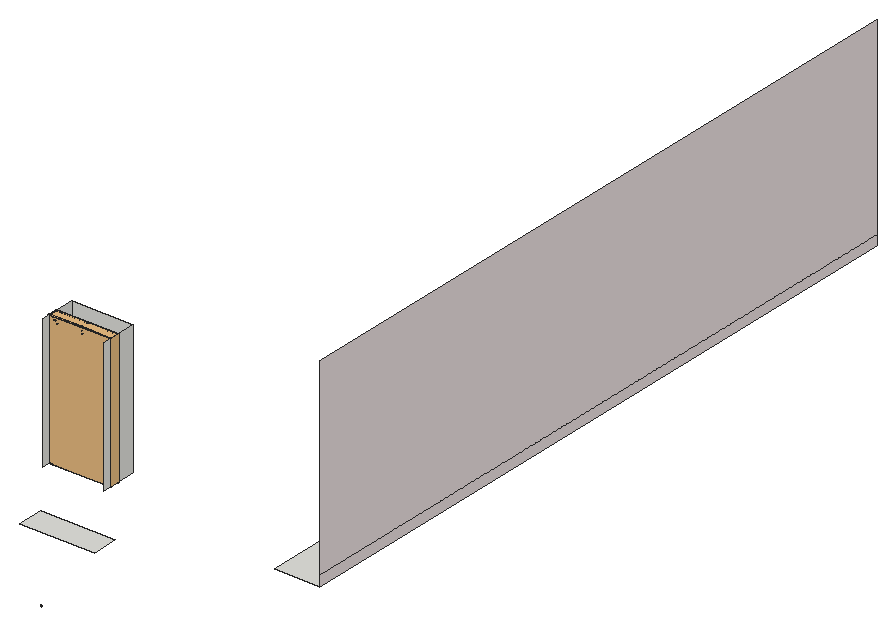
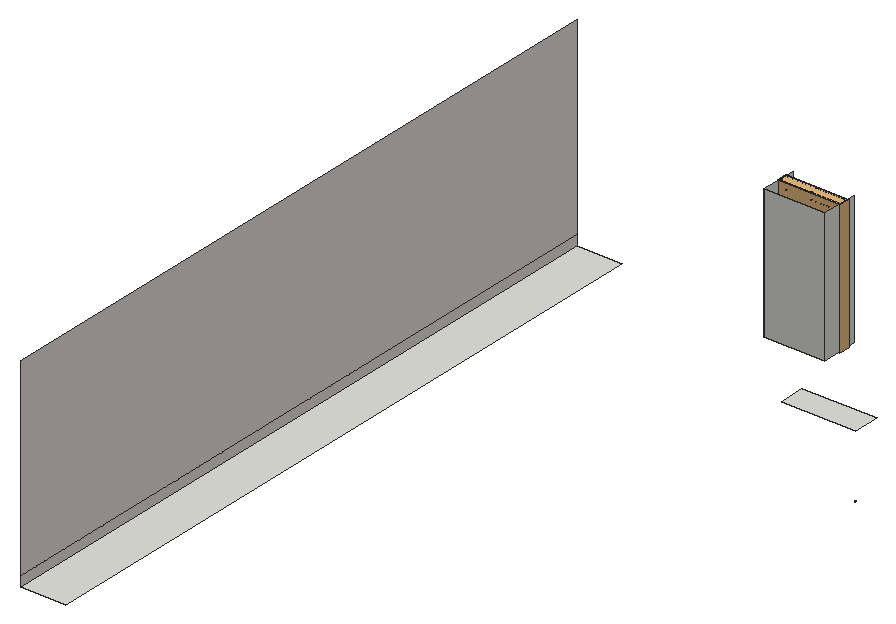
# SketchUp Ruby script. Lengths in inches.
U = 1.inch
M = Sketchup.active_model
def pt(a) = Geom::Point3d.new(a.map { |v| v * U })
def face(e, loops, mat)
  f = e.add_face(loops[0].map { |a| pt(a) })
  loops[1..].each { |l| e.add_face(l.map { |a| pt(a) }).erase! }
  f.material = f.back_material = mat if mat
  f
end
# faces: each face lists its corners as indices into pts; further lists are holes
def faces(e, pts, list, mat = nil) = list.each { |f| face(e, (f[0].is_a?(Array) ? f : [f]).map { |l| l.map { |i| pts[i] } }, mat) }
# xy, xz, yz: faces in a plane at the given z, y or x. An outline is a flat list of corners, or four numbers for a rectangle; further outlines are holes
def ring(l) = l.size == 4 ? [[l[0], l[1]], [l[2], l[1]], [l[2], l[3]], [l[0], l[3]]] : l.each_slice(2).to_a
def flat(e, list, mat, &to3) = list.each { |f| face(e, (f[0].is_a?(Array) ? f : [f]).map { |l| ring(l).map { |u, v| to3.(u, v) } }, mat) }
def xy(e, z, list, mat = nil) = flat(e, list, mat) { |x, y| [x, y, z] }
def xz(e, y, list, mat = nil) = flat(e, list, mat) { |x, z| [x, y, z] }
def yz(e, x, list, mat = nil) = flat(e, list, mat) { |y, z| [x, y, z] }
def lines(e, pts, list) = list.each { |a, b| e.add_line(pt(pts[a]), pt(pts[b])) }
# prism: a flat outline (further loops are holes) pulled along v
def prism(e, loops, v, mat = nil)
  f = face(e, loops, mat); d = Geom::Vector3d.new(v.map { |x| x * U })
  f.pushpull(f.normal.samedirection?(d) ? d.length : -d.length)
end
def box(e, o, s, mat = nil) = prism(e, [[o, [o[0] + s[0], o[1], o[2]], [o[0] + s[0], o[1] + s[1], o[2]], [o[0], o[1] + s[1], o[2]]]], [0, 0, s[2]], mat)
def at(x, y, z, deg = 0) = Geom::Transformation.translation(pt([x, y, z])) * Geom::Transformation.rotation(ORIGIN, Z_AXIS, deg.degrees)
def axes(o, x, y, z) = Geom::Transformation.new([*x, 0, *y, 0, *z, 0, *pt(o).to_a, 1])
def part(name) = M.definitions.add(name)
# library, detail: a bought-in or finely detailed component or shape, given as its bounding box
def library(name, o, s) = part(name).tap { |d| box(d.entities, o, s) }
def detail(e, o, s) = box(e.add_group.entities, o, s)
def put(e, d, t, mat = nil) = e.add_instance(d, t).tap { |i| i.material = mat if mat }
def group(e, t, mat = nil) = e.add_group.tap { |g| g.transformation = t; g.material = mat if mat }.entities
root = M.entities
M.materials.add("Generic\#9").color = [233, 223, 223]
M.materials.add("Material \#0").color = [86, 53, 35]
M.materials.add("Material \#1").color = [140, 140, 140]
c1 = part("3DGeom~19_Defintion")
xy(c1.entities,0,[[-6.28,-215.79,-994.45,-208.55,-13.52,-208.55],[-994.45,-215.79,-994.45,-208.55,-6.28,-215.79],[-6.28,-215.79,-13.52,-208.55,-13.52,0],[-6.28,-215.79,-13.52,0,-6.28,0],[-13.52,0,-13.52,208.55,-6.28,215.79],
  [-13.52,0,-6.28,215.79,-6.28,0],[-994.45,208.55,-6.28,215.79,-13.52,208.55],[-994.45,208.55,-994.45,215.79,-6.28,215.79]],"Material \#0")
p = [[-13.52,-208.55,0],[-994.45,-208.55,0],[-994.45,-207.81,0.07],[-14.25,-207.81,0.07],[-13.52,-208.55,0],[-14.25,-207.81,0.07],
  [-14.25,0,0.07],[-13.52,0,0],[-13.52,208.55,0],[-14.25,207.81,0.07],[-13.52,208.55,0],[-14.25,207.81,0.07],
  [-994.45,207.81,0.07],[-994.45,208.55,0],[-994.45,-207.21,0.27],[-994.45,-207.21,0.27],[-14.86,-207.21,0.27],[-14.86,-207.21,0.27],
  [-14.86,0,0.27],[-14.86,0,0.27],[-14.86,0,0.27],[-14.86,0,0.27],[-14.86,207.21,0.27],[-14.86,207.21,0.27],
  [-994.45,207.21,0.27],[-994.45,207.21,0.27],[-14.86,-207.21,0.27],[-994.45,-207.21,0.27],[-994.45,-206.74,0.6],[-15.33,-206.74,0.6],
  [-14.86,-207.21,0.27],[-15.33,-206.74,0.6],[-15.33,0,0.6],[-14.86,0,0.27],[-14.86,207.21,0.27],[-15.33,206.74,0.6],
  [-14.86,207.21,0.27],[-15.33,206.74,0.6],[-994.45,206.74,0.6],[-994.45,207.21,0.27],[-994.45,-206.4,1.07],[-15.66,-206.4,1.07],
  [-15.66,-206.4,1.07],[-15.66,0,1.07],[-15.66,206.4,1.07],[-15.66,206.4,1.07],[-994.45,206.4,1.07],[-994.45,-206.2,1.68],
  [-15.86,-206.2,1.68],[-15.86,-206.2,1.68],[-15.86,0,1.68],[-15.86,206.2,1.68],[-15.86,206.2,1.68],[-994.45,206.2,1.68],
  [-994.45,-206.13,2.41],[-15.93,-206.13,2.41],[-15.93,-206.13,2.41],[-15.93,0,2.41],[-15.93,206.13,2.41],[-15.93,206.13,2.41],
  [-994.45,206.13,2.41],[-994.45,-206.13,71.16],[-994.45,-206.22,71.59],[-15.79,-206.28,71.53],[-15.79,-206.28,71.53],[-15.84,0,71.59],
  [-15.93,0,71.16],[-15.79,206.28,71.53],[-15.79,206.28,71.53],[-994.45,206.22,71.59],[-994.45,206.13,71.16],[-15.79,-206.28,71.53],
  [-994.45,-206.48,71.84],[-994.45,-206.9,71.93],[-15.16,-206.9,71.93],[-15.79,-206.28,71.53],[-15.79,-206.28,71.53],[-15.16,-206.9,71.93],
  [-15.16,0,71.93],[-994.45,-206.48,71.84],[-15.59,0,71.84],[-15.79,-206.28,71.53],[-15.59,0,71.84],[-15.79,206.28,71.53],
  [-15.16,206.9,71.93],[-15.59,0,71.84],[-15.79,206.28,71.53],[-994.45,206.48,71.84],[-15.79,206.28,71.53],[-15.16,206.9,71.93],
  [-994.45,206.9,71.93],[-994.45,206.48,71.84],[-15.79,206.28,71.53],[-994.45,-227.27,72.01],[5.41,-227.47,72.33],[4.78,-226.84,71.93],
  [4.78,-226.84,71.93],[5.41,-227.47,72.33],[5.21,0,72.01],[-994.45,-226.84,71.93],[-994.45,-227.27,72.01],[5.21,0,72.01],
  [4.78,0,71.93],[4.78,226.84,71.93],[5.21,0,72.01],[5.21,0,72.01],[5.41,227.47,72.33],[4.78,226.84,71.93],
  [5.41,227.47,72.33],[-994.45,227.27,72.01],[-994.45,227.27,72.01],[-994.45,226.84,71.93],[-994.45,-227.27,72.01],[-994.45,-227.53,72.27],
  [5.41,-227.47,72.33],[5.41,-227.47,72.33],[5.47,0,72.27],[5.21,0,72.01],[5.41,227.47,72.33],[5.41,227.47,72.33],
  [-994.45,227.53,72.27],[-994.45,227.27,72.01],[-994.45,-227.61,72.7],[-994.45,-227.61,74.4375],[-994.45,-227.61,74.4375],[5.55,-227.61,74.4375],
  [5.55,-227.61,74.4375],[5.55,0,74.4375],[5.55,0,72.7],[5.55,227.61,74.4375],[5.55,227.61,74.4375],[-994.45,227.61,74.4375],
  [-994.45,227.61,74.4375],[-994.45,227.61,72.7]]
faces(c1.entities,p,[[0,1,2],[2,3,0],[4,5,6],[6,7,4],[8,7,6],[6,9,8],[10,11,12],[12,13,10],
  [3,2,14],[15,16,3],[5,17,18],[19,6,5],[9,6,20],[21,22,9],[11,23,24],[25,12,11],
  [26,27,28],[28,29,26],[30,31,32],[32,33,30],[34,33,32],[32,35,34],[36,37,38],[38,39,36],
  [29,28,40],[40,41,29],[31,42,43],[43,32,31],[35,32,43],[43,44,35],[37,45,46],[46,38,37],
  [41,40,47],[47,48,41],[42,49,50],[50,43,42],[44,43,50],[50,51,44],[45,52,53],[53,46,45],
  [48,47,54],[54,55,48],[49,56,57],[57,50,49],[51,50,57],[57,58,51],[52,59,60],[60,53,52],
  [61,62,63],[64,65,66],[66,65,67],[68,69,70],[71,72,73],[73,74,75],[76,77,78],[62,79,63],
  [78,80,76],[81,82,65],[83,80,78],[78,84,83],[65,85,86],[68,87,69],[88,89,90],[90,91,92],
  [93,94,95],[96,97,98],[95,99,100],[101,102,96],[103,102,104],[105,106,103],[107,108,109],[110,111,107],
  [112,113,114],[115,116,117],[117,116,118],[119,120,121],[114,122,123],[124,125,114],[113,122,114],[115,126,127],
  [127,128,115],[115,128,116],[118,128,127],[127,129,118],[116,128,118],[119,130,131],[132,133,119],[119,133,120]],"Material \#0")
c2 = part("3DGeom~15_Defintion")
xy(c2.entities,0,[[-961.58,-251.9,-958.5,-248.8125,-961.58,-237.8],[-961.58,-251.9,28.8,-248.8125,-958.5,-248.8125],[-961.58,-251.9,36.25,-251.9,28.8,-248.8125],[36.25,-251.9,19.98,-239.99,28.8,-248.8125],[36.25,-251.9,22.16,-237.8,19.98,-239.99],
  [-958.5,-248.8125,-958.5,-237.8,-961.58,-237.8],[19.98,-239.99,22.16,-237.8,3.36,-223.37],[-958.5,-237.8,-958.5,-223.37,-961.58,-220.28],[-961.58,-237.8,-958.5,-237.8,-961.58,-220.28],[22.16,-237.8,4.64,-220.28,3.36,-223.37],
  [-958.5,-223.37,4.64,-220.28,-961.58,-220.28],[-958.5,-223.37,3.36,-223.37,4.64,-220.28],[5.29,-219.63,8.375,-218.35,5.29,0],[8.375,-218.35,8.375,0,5.29,0],[5.29,0,8.375,0,5.29,219.63],
  [8.375,0,8.375,218.35,5.29,219.63],[8.375,218.35,22.8125,237.15,5.29,219.63],[-961.58,220.28,-958.5,223.37,-961.58,237.8],[-961.58,220.28,3.36,223.37,-958.5,223.37],[-961.58,220.28,4.64,220.28,3.36,223.37],
  [4.64,220.28,19.98,239.99,3.36,223.37],[4.64,220.28,22.16,237.8,19.98,239.99],[-958.5,223.37,-958.5,237.8,-961.58,237.8],[-958.5,237.8,-958.5,248.8125,-961.58,251.9],[-961.58,237.8,-958.5,237.8,-961.58,251.9],
  [22.16,237.8,28.8,248.8125,19.98,239.99],[22.16,237.8,36.25,251.9,28.8,248.8125],[-958.5,248.8125,36.25,251.9,-961.58,251.9],[-958.5,248.8125,28.8,248.8125,36.25,251.9]],"Material \#0")
xy(c2.entities,7.48,[[-962.79,-238.36,23.37,-238.36,-962.79,-219.67],[23.37,-238.36,4.67,-219.67,-962.79,-219.67],[23.37,-238.36,23.37,0,4.67,-219.67],[4.67,-219.67,23.37,0,4.67,0],[23.37,0,23.37,238.36,4.67,219.67],
  [4.67,0,23.37,0,4.67,219.67],[-962.79,219.67,23.37,238.36,-962.79,238.36],[-962.79,219.67,4.67,219.67,23.37,238.36]],"Material \#0")
xy(c2.entities,63.5625,[[-962.79,-238.36,-962.79,-219.67,4.67,-219.67],[-962.79,-238.36,4.67,-219.67,23.37,-238.36],[23.37,-238.36,4.67,-219.67,23.37,0],[4.67,-219.67,4.67,0,23.37,0],[23.37,0,4.67,219.67,23.37,238.36],
  [4.67,0,4.67,219.67,23.37,0],[-962.79,219.67,-962.79,238.36,4.67,219.67],[4.67,219.67,-962.79,238.36,23.37,238.36]],"Material \#0")
xy(c2.entities,69.64,[[-962.79,-219.62,4.63,-219.62,-962.79,-200.32],[4.63,-219.62,-14.68,-200.32,-962.79,-200.32],[4.63,-219.62,4.63,0,-14.68,-200.32],[-14.68,-200.32,4.63,0,-14.68,0],[-14.68,0,4.63,0,-14.68,200.32],
  [4.63,0,4.63,219.62,-14.68,200.32],[-962.79,200.32,-14.68,200.32,4.63,219.62],[-962.79,200.32,4.63,219.62,-962.79,219.62]],"Material \#0")
xy(c2.entities,71.04,[[-961.58,-251.9,-958.5,-248.8125,28.8,-248.8125],[-961.58,-251.9,-961.58,-237.8,-958.5,-248.8125],[-961.58,-251.9,28.8,-248.8125,36.25,-251.9],[36.25,-251.9,19.98,-239.99,22.16,-237.8],[36.25,-251.9,28.8,-248.8125,19.98,-239.99],
  [-958.5,-248.8125,-961.58,-237.8,-958.5,-237.8],[19.98,-239.99,3.36,-223.37,22.16,-237.8],[-958.5,-237.8,-961.58,-220.28,-958.5,-223.37],[-961.58,-237.8,-961.58,-220.28,-958.5,-237.8],[22.16,-237.8,3.36,-223.37,4.64,-220.28],
  [-958.5,-223.37,-961.58,-220.28,4.64,-220.28],[-958.5,-223.37,4.64,-220.28,3.36,-223.37],[5.29,-219.63,5.29,0,8.375,-218.35],[8.375,-218.35,5.29,0,8.375,0],[5.29,0,5.29,219.63,8.375,0],
  [8.375,0,5.29,219.63,8.375,218.35],[8.375,218.35,5.29,219.63,22.8125,237.15],[-961.58,220.28,-958.5,223.37,3.36,223.37],[-961.58,220.28,-961.58,237.8,-958.5,223.37],[-961.58,220.28,3.36,223.37,4.64,220.28],
  [4.64,220.28,3.36,223.37,19.98,239.99],[4.64,220.28,19.98,239.99,22.16,237.8],[-958.5,223.37,-961.58,237.8,-958.5,237.8],[-958.5,237.8,-961.58,251.9,-958.5,248.8125],[-961.58,237.8,-961.58,251.9,-958.5,237.8],
  [22.16,237.8,19.98,239.99,28.8,248.8125],[22.16,237.8,28.8,248.8125,36.25,251.9],[-958.5,248.8125,-961.58,251.9,36.25,251.9],[-958.5,248.8125,36.25,251.9,28.8,248.8125]],"Material \#0")
xz(c2.entities,-238.36,[[-962.79,63.5625,23.37,63.5625,23.37,72.07],[-962.79,63.5625,23.37,72.07,-962.79,72.07]],"Material \#0")
xz(c2.entities,-219.67,[[-962.79,7.48,4.67,7.48,-962.79,63.5625],[4.67,7.48,4.67,63.5625,-962.79,63.5625]],"Material \#0")
xz(c2.entities,219.67,[[-962.79,7.48,-962.79,63.5625,4.67,7.48],[4.67,7.48,-962.79,63.5625,4.67,63.5625]],"Material \#0")
xz(c2.entities,238.36,[[-962.79,63.5625,-962.79,72.07,23.37,72.07],[-962.79,63.5625,23.37,72.07,23.37,63.5625]],"Material \#0")
yz(c2.entities,4.67,[[-219.67,7.48,0,7.48,-219.67,63.5625],[0,7.48,0,63.5625,-219.67,63.5625],[0,7.48,219.67,63.5625,0,63.5625],[0,7.48,219.67,7.48,219.67,63.5625]],"Material \#0")
yz(c2.entities,23.37,[[-238.36,63.5625,0,63.5625,-238.36,72.07],[0,63.5625,0,72.07,-238.36,72.07],[0,63.5625,238.36,63.5625,238.36,72.07],[0,63.5625,238.36,72.07,0,72.07]],"Material \#0")
p = [[36.9,-251.24,0],[37.21,0,-0.16],[34.125,0,-0.14],[36.9,251.24,0],[33.83,243.81,0.02],[33.83,-243.8,0.02],
  [22.8125,-237.15,0],[24.99,-234.97,-0.01],[5.375,-220.37,0],[23.37,-238.36,7.48],[4.67,-219.67,7.48],[4.67,-219.67,7.48],
  [23.37,-238.36,7.48],[23.37,-238.36,0],[4.67,-219.67,7.48],[23.37,-238.36,0],[5.375,-220.37,0],[5.375,-220.37,0],
  [23.37,-238.36,0],[5.29,-219.63,0],[8.375,-218.35,0],[-15.36,-199.64,1.62],[4.67,-219.67,7.48],[5.375,-220.37,0],
  [-13.8,-201.19,0.06],[5.375,-220.37,0],[5.375,-220.37,0],[-14.84,-200.15,0.58],[5.375,-220.37,0],[-13.8,-201.19,0.06],
  [-6.08,-208.92,0],[5.375,-220.37,0],[-13.8,-201.19,0.06],[-6.08,-208.92,0],[-13.8,-201.19,0.06],[5.375,-220.37,0],
  [-6.08,-208.92,0],[-13.8,-201.19,0.06],[-13.09,-201.91,0],[-6.08,-208.92,0],[-13.09,-201.91,0],[-13.8,-201.19,0.06],
  [-15.36,199.64,1.62],[4.67,219.67,7.48],[5.375,220.37,0],[-13.8,201.19,0.06],[5.375,220.37,0],[5.375,220.37,0],
  [4.67,219.67,7.48],[-14.84,200.15,0.58],[5.375,220.37,0],[-13.8,201.19,0.06],[-6.08,208.92,0],[-13.09,201.91,0],
  [-13.8,201.19,0.06],[-6.08,208.92,0],[-13.8,201.19,0.06],[5.375,220.37,0],[-6.08,208.92,0],[5.375,220.37,0],
  [-13.8,201.19,0.06],[-6.08,208.92,0],[-13.8,201.19,0.06],[-13.09,201.91,0],[8.375,218.35,0],[24.99,234.97,-0.01],
  [22.8125,237.15,0],[23.37,238.36,7.48],[23.37,238.36,0],[23.37,238.36,0],[5.375,220.37,0],[5.375,220.37,0],
  [23.37,238.36,7.48],[4.67,219.67,7.48],[5.375,220.37,0],[23.37,238.36,0],[23.37,238.36,7.48],[-13.8,-201.19,0.06],
  [-14.84,-200.15,0.58],[-14.38,-200.61,0.26],[-13.8,-201.19,0.06],[-13.8,-201.19,0.06],[-14.38,-200.61,0.26],[-13.8,201.19,0.06],
  [-14.84,200.15,0.58],[-13.8,201.19,0.06],[-14.38,200.61,0.26],[-14.38,200.61,0.26],[-13.8,201.19,0.06],[4.63,-219.62,69.64],
  [4.63,-219.62,69.64],[-15.42,-199.57,9.43],[-15.36,-199.64,1.62],[-15.16,-199.83,1.04],[-15.16,-199.83,1.04],[-15.16,199.83,1.04],
  [-15.36,199.64,1.62],[-15.16,199.83,1.04],[-15.42,199.57,9.43],[4.63,219.62,69.64],[4.67,219.67,7.48],[4.63,219.62,69.64],
  [4.63,-219.62,69.64],[4.67,-219.67,63.5625],[4.67,-219.67,63.5625],[4.67,-219.67,7.48],[-15.28,-199.71,69.25],[4.63,-219.62,69.64],
  [-15.42,-199.57,9.43],[-15.28,-199.71,69.25],[-15.42,-199.57,2.34],[-15.42,-199.57,2.34],[-15.42,199.57,2.34],[-15.42,199.57,9.43],
  [-15.28,199.71,69.25],[-15.28,199.71,69.25],[4.63,219.62,69.64],[4.63,219.62,69.64],[4.67,219.67,63.5625],[4.67,219.67,63.5625],
  [-15.42,199.57,2.34],[4.67,-219.67,63.5625],[4.63,-219.62,69.64],[4.67,219.67,7.48],[4.67,219.67,63.5625],[4.63,219.62,69.64],
  [4.63,-219.62,69.64],[-15.28,-199.71,69.25],[-15.28,-199.71,69.25],[-15.42,-199.57,48.99],[-15.42,-199.57,48.99],[-15.28,-199.71,69.25],
  [-15.42,199.57,48.99],[-15.28,199.71,69.25],[-15.28,199.71,69.25],[-15.42,199.57,48.99],[4.63,219.62,69.64],[4.63,-219.62,69.64],
  [23.37,-238.36,72.07],[4.67,-219.67,63.5625],[4.67,-219.67,63.5625],[23.37,-238.36,63.5625],[23.37,-238.36,72.07],[4.67,-219.67,63.5625],
  [5.24,-220.23,70.03],[23.37,-238.36,72.07],[23.37,-238.36,63.5625],[4.67,-219.67,63.5625],[4.67,-219.67,63.5625],[4.63,-219.62,69.64],
  [4.63,219.62,69.64],[23.37,238.36,72.07],[4.67,219.67,63.5625],[4.67,219.67,63.5625],[5.24,220.23,70.03],[4.63,219.62,69.64],
  [23.37,238.36,63.5625],[4.67,219.67,63.5625],[4.67,219.67,63.5625],[23.37,238.36,63.5625],[23.37,238.36,72.07],[4.67,219.67,63.5625],
  [23.37,238.36,72.07],[4.63,-219.62,69.64],[-14.68,-200.32,69.64],[-15.28,-199.71,69.25],[-15.28,-199.71,69.25],[-14.68,-200.32,69.64],
  [4.63,-219.62,69.64],[-15.28,199.71,69.25],[-14.68,200.32,69.64],[4.63,219.62,69.64],[4.63,219.62,69.64],[-14.68,200.32,69.64],
  [4.63,-219.62,69.64],[5.24,-220.23,70.03],[23.37,-238.36,72.07],[4.63,219.62,69.64],[5.24,220.23,70.03],[5.375,-220.37,72.07],
  [5.375,-220.37,72.07],[23.37,-238.36,72.07],[5.375,220.37,72.07],[23.37,238.36,72.07],[5.375,220.37,72.07],[33.83,-243.8,71.03],
  [36.9,-251.24,71.04],[22.8125,-237.15,71.04],[34.125,0,71.19],[37.21,0,71.2],[24.99,-234.97,71.05],[5.29,-219.63,71.04],
  [8.375,-218.35,71.04],[33.83,243.81,71.03],[36.9,251.24,71.04],[22.8125,237.15,71.04],[24.99,234.97,71.05],[8.375,218.35,71.04]]
faces(c2.entities,p,[[0,1,2],[1,3,4],[4,2,1],[2,5,0],[6,0,5],[5,7,6],[8,9,10],[11,12,13],
  [14,15,16],[17,18,9],[19,6,7],[7,20,19],[21,22,23],[24,21,25],[26,10,27],[28,27,29],
  [30,31,32],[33,34,35],[36,37,38],[39,40,41],[42,43,44],[45,42,46],[47,48,49],[50,49,51],
  [52,53,54],[55,56,57],[58,59,60],[61,62,63],[64,65,66],[43,67,68],[43,69,70],[71,72,73],
  [74,75,76],[3,66,65],[65,4,3],[77,78,21],[27,79,80],[81,82,78],[83,84,42],[85,86,84],
  [49,87,88],[10,89,27],[90,91,27],[92,93,27],[91,92,27],[78,94,21],[84,95,42],[96,97,49],
  [98,96,49],[99,98,49],[100,101,49],[21,102,103],[21,104,105],[21,106,107],[21,108,109],[91,110,92],
  [21,111,108],[42,112,113],[42,113,114],[42,115,116],[42,117,118],[42,119,43],[98,120,96],[10,121,122],
  [123,124,125],[126,127,91],[128,129,91],[108,130,131],[113,132,133],[134,135,98],[136,134,98],[137,138,139],
  [140,141,142],[143,142,144],[145,146,147],[148,144,149],[150,151,152],[153,154,155],[151,156,157],[158,159,160],
  [161,162,154],[163,164,165],[166,167,168],[169,170,171],[172,173,134],[174,175,176],[177,178,151],[142,179,144],
  [175,180,181],[178,182,151],[183,184,154],[185,186,187],[186,185,188],[188,189,186],[187,190,185],[190,187,191],
  [191,192,190],[189,188,193],[193,194,189],[195,196,197],[196,195,194],[194,193,196]],"Material \#0")
c3 = part("3DGeom~22_Defintion")
xz(c3.entities,-210.625,[[-1016.13,2.47,-1016.13,9.96,-16.28,2.47],[-16.28,2.47,-1016.13,9.96,-16.28,9.96],[-1016.13,9.96,-1016.13,51.7,-16.28,51.7],[-1016.13,9.96,-16.28,51.7,-16.28,9.96],[-1016.13,51.7,-1016.13,72.71,-16.28,51.7]],"Material \#0")
xz(c3.entities,210.625,[[-1016.13,2.47,-16.28,2.47,-1016.13,9.96],[-16.28,2.47,-16.28,9.96,-1016.13,9.96],[-1016.13,9.96,-16.28,51.7,-1016.13,51.7],[-1016.13,9.96,-16.28,9.96,-16.28,51.7],[-1016.13,51.7,-16.28,51.7,-1016.13,72.71]],"Material \#0")
yz(c3.entities,-16.28,[[-210.625,2.47,-210.625,9.96,0,9.96],[-210.625,2.47,0,9.96,0,2.47],[0,2.47,0,9.96,210.625,2.47],[210.625,2.47,0,9.96,210.625,9.96],[-210.625,9.96,-210.625,51.7,0,51.7],
  [-210.625,9.96,0,51.7,0,9.96],[0,9.96,0,51.7,210.625,9.96],[210.625,9.96,0,51.7,210.625,51.7],[-210.625,51.7,0,72.71,0,51.7],[0,51.7,0,72.71,210.625,51.7]],"Material \#0")
p = [[-1016.13,-210.625,72.71],[-16.13,-210.77,73.09],[-16.28,-210.625,51.7],[-16.28,-210.625,51.7],[-16.13,-210.77,73.09],[-16.28,0,72.71],
  [-16.13,210.77,73.09],[-16.28,210.625,51.7],[-16.28,210.625,51.7],[-16.13,210.77,73.09],[-1016.13,210.625,72.71]]
faces(c3.entities,p,[[0,1,2],[3,4,5],[5,6,7],[8,9,10]],"Material \#0")
c4 = library("3DGeom~16_Defintion",[-962.62,-252.34,-11.22],[1000,504.68,93.46])
c5 = part("3DGeom~17_Defintion")
yz(c5.entities,-1908.8,[[-436.03,-21.87,-436.73,-21.5,-435.91,-21.83],[436.03,-21.87,435.91,-21.83,436.73,-21.5],[-435.91,-21.83,-436.73,-21.5,-436.15,-21.125],[-435.91,-21.83,-436.15,-21.125,-435.87,-21.72],[435.91,-21.83,435.87,-21.72,436.15,-21.125],
  [435.91,-21.83,436.15,-21.125,436.73,-21.5],[-436.73,-21.5,-484.73,-21.37,-436.15,-1.11],[-471.46,-21.5,-484.73,-21.37,-436.73,-21.5],[-477.2,-21.5,-484.73,-21.37,-471.46,-21.5],[-481.82,-21.5,-484.73,-21.37,-477.2,-21.5],
  [-436.73,-21.5,-436.15,-1.11,-436.15,-21.125],[436.73,-21.5,436.15,-21.125,471.46,-21.5],[471.46,-21.5,436.15,-21.125,477.2,-21.5],[477.2,-21.5,436.15,-21.125,499.98,-0.85],[477.2,-21.5,499.98,-0.85,481.82,-21.5],
  [481.82,-21.5,487.35,-21,484.73,-21.37],[481.82,-21.5,491.8,-19.52,487.35,-21],[481.82,-21.5,497.64,-13.67,491.8,-19.52],[481.82,-21.5,499.98,-0.85,497.64,-13.67],[-484.73,-21.37,-498.5,-11.58,-499.84,-0.37],
  [-484.73,-21.37,-499.84,-0.37,-499.4,-0.5],[-484.73,-21.37,-499.4,-0.5,-436.15,-1.11],[-484.73,-21.37,-493.63,-18.42,-498.5,-11.58],[-484.73,-21.37,-489.71,-20.375,-493.63,-18.42],[-484.73,-21.37,-487.35,-21,-489.71,-20.375],
  [436.15,-21.125,436.15,-1.11,436.73,-0.74],[436.15,-21.125,436.73,-0.74,499.98,-0.85],[487.35,-21,491.8,-19.52,489.71,-20.375],[-489.71,-20.375,-491.8,-19.52,-493.63,-18.42],[491.8,-19.52,495.21,-17.08,493.63,-18.42],
  [491.8,-19.52,497.64,-13.67,495.21,-17.08],[-493.63,-18.42,-496.54,-15.5,-498.5,-11.58],[-493.63,-18.42,-495.21,-17.08,-496.54,-15.5],[495.21,-17.08,497.64,-13.67,496.54,-15.5],[-496.54,-15.5,-497.64,-13.67,-498.5,-11.58],
  [497.64,-13.67,499.125,-9.22,498.5,-11.58],[497.64,-13.67,499.625,-3.69,499.125,-9.22],[497.64,-13.67,499.98,-0.85,499.625,-3.69],[-498.5,-11.58,-499.625,-3.69,-499.84,-0.37],[-498.5,-11.58,-499.5,-6.6,-499.625,-3.69],
  [-498.5,-11.58,-499.125,-9.22,-499.5,-6.6],[499.125,-9.22,499.625,-3.69,499.5,-6.6],[-499.625,-3.69,-499.98,-0.85,-500,-0.52],[-499.625,-3.69,-500,-0.52,-499.84,-0.37],[-436.15,-1.11,-499.4,-0.5,-471.46,-0.74],
  [-436.15,-1.11,-471.46,-0.74,-436.73,-0.74],[-436.15,-1.11,-436.73,-0.74,-435.91,-0.41],[-436.15,-1.11,-435.91,-0.41,-435.87,-0.52],[436.15,-1.11,435.87,-0.52,435.91,-0.41],[436.15,-1.11,435.91,-0.41,436.73,-0.74],
  [499.98,-0.85,436.73,-0.74,471.46,-0.74],[499.98,-0.85,471.46,-0.74,499.4,-0.5],[499.98,-0.85,499.4,-0.5,499.96,-0.41],[499.98,-0.85,499.96,-0.41,500,-0.52],[-436.73,-0.74,-436.03,-0.37,-435.91,-0.41],
  [436.73,-0.74,435.91,-0.41,436.03,-0.37],[-500,-0.52,-499.96,-0.41,-499.84,-0.37],[499.4,-0.5,499.84,-0.37,499.96,-0.41],[-499.84,141.21,-499.96,141.25,-499.4,141.35],[-436.03,141.21,-436.73,141.59,-435.91,141.25],
  [436.03,141.21,435.91,141.25,436.73,141.59],[499.84,141.21,484.73,162.21,498.5,152.42],[499.84,141.21,499.4,141.35,484.73,162.21],[499.84,141.21,498.5,152.42,499.625,144.53],[499.84,141.21,499.625,144.53,500,141.37],
  [499.84,141.21,500,141.37,499.96,141.25],[-499.96,141.25,-500,141.37,-499.98,141.69],[-499.96,141.25,-499.98,141.69,-499.4,141.35],[-435.91,141.25,-436.73,141.59,-436.15,141.96],[-435.91,141.25,-436.15,141.96,-435.87,141.37],
  [435.91,141.25,435.87,141.37,436.15,141.96],[435.91,141.25,436.15,141.96,436.73,141.59],[-499.4,141.35,-499.98,141.69,-471.46,141.59],[499.4,141.35,436.15,141.96,484.73,162.21],[499.4,141.35,471.46,141.59,436.15,141.96],
  [500,141.37,499.625,144.53,499.98,141.69],[-436.73,141.59,-499.98,141.69,-436.15,161.97],[-471.46,141.59,-499.98,141.69,-436.73,141.59],[-436.73,141.59,-436.15,161.97,-436.15,141.96],[436.73,141.59,436.15,141.96,471.46,141.59],
  [-499.98,141.69,-477.2,162.34,-436.15,161.97],[-499.98,141.69,-481.82,162.34,-477.2,162.34],[-499.98,141.69,-497.64,154.51,-481.82,162.34],[-499.98,141.69,-499.625,144.53,-497.64,154.51],[436.15,141.96,436.15,161.97,436.73,162.34],
  [436.15,141.96,436.73,162.34,484.73,162.21],[-499.625,144.53,-499.125,150.07,-497.64,154.51],[-499.625,144.53,-499.5,147.44,-499.125,150.07],[499.625,144.53,498.5,152.42,499.5,147.44],[499.5,147.44,498.5,152.42,499.125,150.07],
  [-499.125,150.07,-498.5,152.42,-497.64,154.51],[498.5,152.42,484.73,162.21,493.63,159.26],[498.5,152.42,493.63,159.26,496.54,156.34],[498.5,152.42,496.54,156.34,497.64,154.51],[-497.64,154.51,-491.8,160.36,-481.82,162.34],
  [-497.64,154.51,-495.21,157.92,-491.8,160.36],[-497.64,154.51,-496.54,156.34,-495.21,157.92],[496.54,156.34,493.63,159.26,495.21,157.92],[-495.21,157.92,-493.63,159.26,-491.8,160.36],[493.63,159.26,484.73,162.21,489.71,161.22],
  [493.63,159.26,489.71,161.22,491.8,160.36],[-491.8,160.36,-487.35,161.84,-481.82,162.34],[-491.8,160.36,-489.71,161.22,-487.35,161.84],[489.71,161.22,484.73,162.21,487.35,161.84],[-487.35,161.84,-484.73,162.21,-481.82,162.34],
  [-436.15,161.97,-477.2,162.34,-471.46,162.34],[-436.15,161.97,-471.46,162.34,-436.73,162.34],[-436.15,161.97,-436.73,162.34,-435.91,162.68],[-436.15,161.97,-435.91,162.68,-435.87,162.56],[436.15,161.97,435.87,162.56,435.91,162.68],
  [436.15,161.97,435.91,162.68,436.73,162.34],[484.73,162.21,436.73,162.34,471.46,162.34],[484.73,162.21,471.46,162.34,477.2,162.34],[484.73,162.21,477.2,162.34,481.82,162.34],[-436.73,162.34,-436.03,162.72,-435.91,162.68],
  [436.73,162.34,435.91,162.68,436.03,162.72]],"Material \#0")
c6 = part("3DGeom~18_Defintion")
xz(c6.entities,-241.71,[[-976.3,0,23.7,0,23.7,7.58],[-976.3,0,23.7,7.58,-976.3,7.58]],"Material \#0")
xz(c6.entities,241.71,[[-976.3,0,-976.3,7.58,23.7,7.58],[-976.3,0,23.7,7.58,23.7,0]],"Material \#0")
yz(c6.entities,23.7,[[-241.71,0,0,0,-241.71,7.58],[0,0,0,7.58,-241.71,7.58],[0,0,241.71,0,241.71,7.58],[0,0,241.71,7.58,0,7.58]],"Material \#0")
c7 = part("3DGeom~20_Defintion")
xy(c7.entities,0,[[-976.3,-241.71,-976.3,-223.46,23.7,-241.71],[23.7,-241.71,-976.3,-223.46,5.45,-223.46],[23.7,-241.71,5.45,-223.46,5.45,0],[23.7,-241.71,5.45,0,23.7,0],[-976.3,-223.46,-976.3,-211.85,5.45,-223.46],
  [5.45,-223.46,-976.3,-211.85,-6.16,-211.85],[5.45,-223.46,-6.16,-211.85,-6.16,0],[5.45,-223.46,-6.16,0,5.45,0],[-6.16,0,-6.16,211.85,5.45,223.46],[-6.16,0,5.45,223.46,5.45,0],
  [5.45,0,23.7,241.71,23.7,0],[5.45,0,5.45,223.46,23.7,241.71],[-976.3,211.85,-976.3,223.46,5.45,223.46],[-976.3,211.85,5.45,223.46,-6.16,211.85],[-976.3,223.46,-976.3,241.71,23.7,241.71],
  [-976.3,223.46,23.7,241.71,5.45,223.46]],"Material \#0")
xy(root,90.9375,[[340.78,194.8125,384.72,210.0625]])
xy(root,120,[[491.875,194.8125,518.6875,607.4375]])
xz(root,201.11,[[348.54,46.74,348.55,46.74,348.52,46.875],[348.55,46.74,348.54,46.88,348.52,46.875],[347.91,46.81,347.95,46.83,347.9375,46.84],[347.95,46.83,347.97,46.86,347.9375,46.84],[347.95,46.83,347.98,46.85,347.97,46.86],
  [347.98,46.85,348,46.89,347.97,46.86],[347.98,46.85,348.01,46.88,348,46.89],[348.52,46.875,348.54,46.88,348.49,47],[348.01,46.88,348.02,46.92,348,46.89],[348.01,46.88,348.03,46.92,348.02,46.92],
  [348.54,46.88,348.5,47,348.49,47],[348.02,46.92,348.03,46.92,348.04,46.96],[348.03,46.92,348.05,46.95,348.04,46.96],[348.05,46.95,348.05,47,348.04,46.96],[348.05,46.95,348.0625,47,348.05,47],
  [348.05,47,348.0625,47,348.05,47.04],[348.0625,47,348.06,47.04,348.05,47.04],[348.06,47.04,348.0625,47.09,348.05,47.08],[348.05,47.08,348.0625,47.09,348.04,47.12],[348.0625,47.09,348.05,47.13,348.04,47.12],
  [348.04,47.12,348.05,47.13,348.02,47.16],[348.05,47.13,348.03,47.17,348.02,47.16],[348.02,47.16,348.03,47.17,348,47.19],[348.03,47.17,348.01,47.2,348,47.19],[348,47.19,348.01,47.2,347.97,47.22],
  [348.01,47.2,347.98,47.23,347.97,47.22],[348.37,47.21,348.38,47.22,348.28,47.3],[347.97,47.22,347.98,47.23,347.9375,47.24],[348.38,47.22,348.29,47.3125,348.28,47.3],[347.98,47.23,347.95,47.25,347.9375,47.24],
  [347.9375,47.24,347.95,47.25,347.9,47.26],[348.28,47.3,348.29,47.3125,348.18,47.375],[348.29,47.3125,348.1875,47.39,348.18,47.375],[348.18,47.375,348.1875,47.39,348.07,47.43],[348.1875,47.39,348.08,47.44,348.07,47.43],
  [348.07,47.43,348.08,47.44,347.95,47.46],[348.08,47.44,347.95,47.47,347.95,47.46]],"Material \#1")
xz(root,216.25,[[354.24,126,390.67,204.625]])
yz(root,354.24,[[194.75,126,216.25,204.625]])
yz(root,390.67,[[194.75,126,216.25,204.625]])
yz(root,518.6875,[[194.8125,120,607.4375,120,607.4375,126,194.75,126],[194.75,126,607.4375,240]],"Generic\#9")
put(root,c1,axes([372.33,204.75,201.6875],[0,0,0.07611],[0.07154,0,0],[0,-0.06445,0]),"Material \#0")
put(root,c2,axes([372.33,204.75,201.6875],[0,0,0.07861],[0.07389,0,0],[0,-0.06657,0]),"Material \#0")
put(root,c3,axes([372.33,204.75,201.6875],[0,0,0.07448],[0.07002,0,0],[0,-0.06308,0]),"Material \#0")
put(root,c4,axes([372.33,204.75,201.6875],[0,0,0.07862],[0.07391,0,0],[0,-0.06658,0]),"Material \#0")
put(root,c5,axes([372.33,204.75,201.6875],[0,0,0.03965],[0.03727,0,0],[0,-0.03358,0]),"Material \#0")
put(root,c6,axes([372.33,204.75,201.6875],[0,0,0.07752],[0.07287,0,0],[0,-0.06565,0]),"Material \#0")
put(root,c7,axes([372.33,204.75,201.6875],[0,0,0.07752],[0.07287,0,0],[0,-0.06565,0]),"Material \#0")
